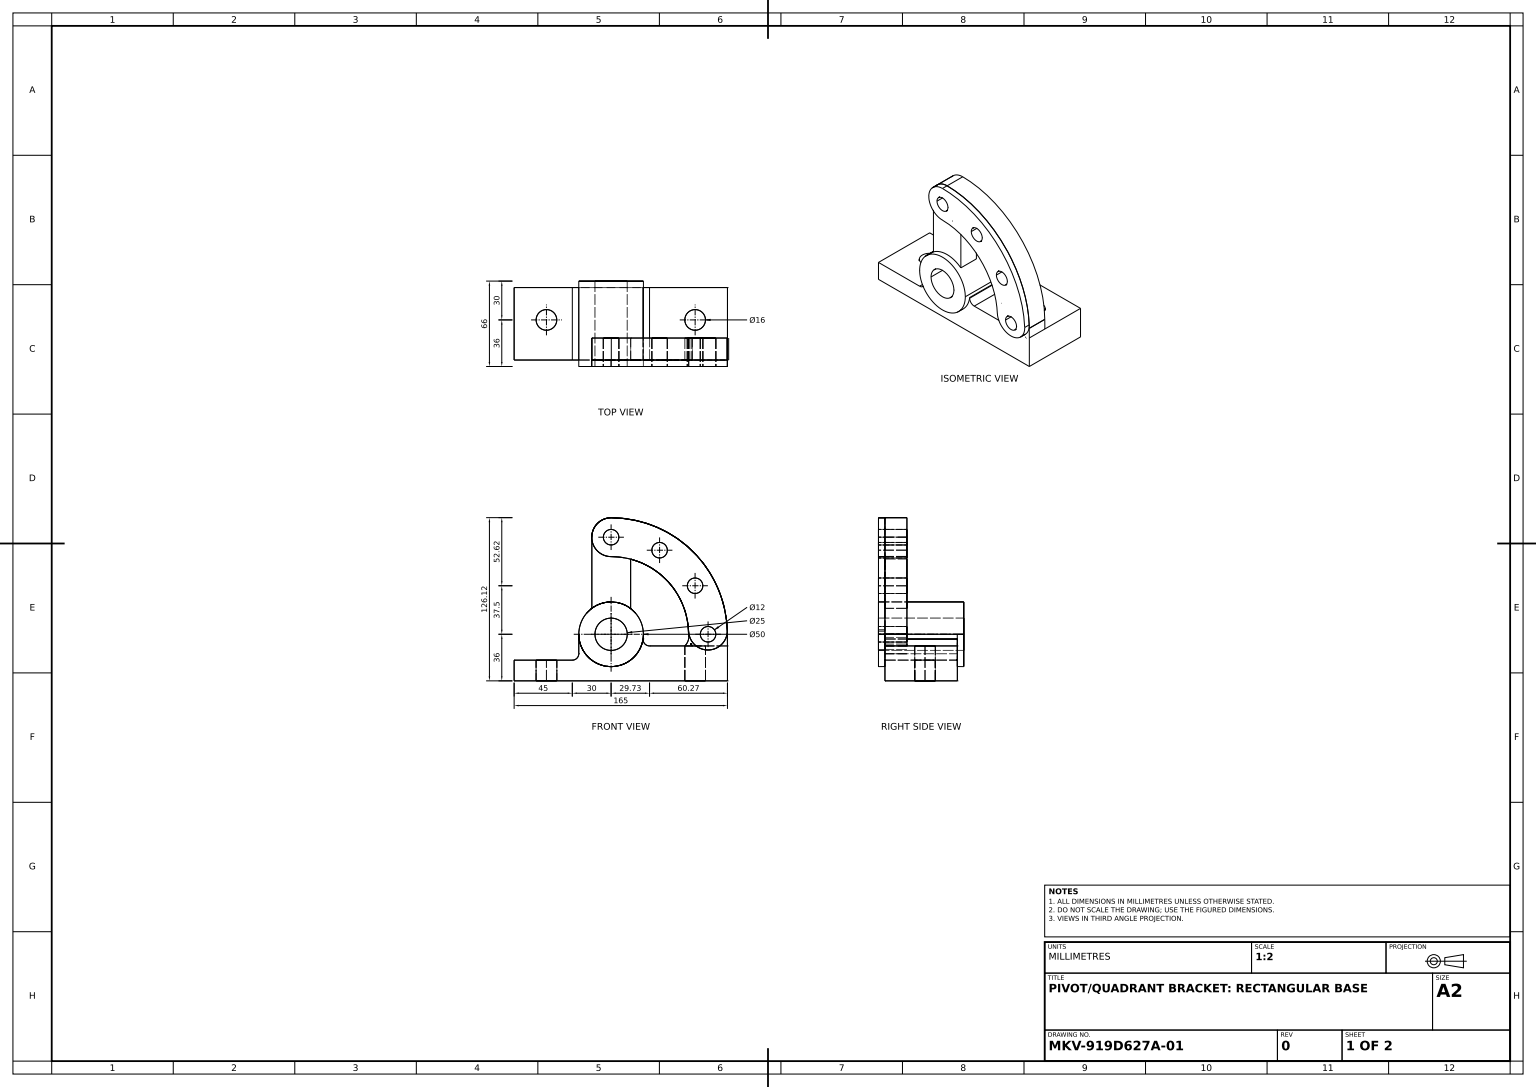
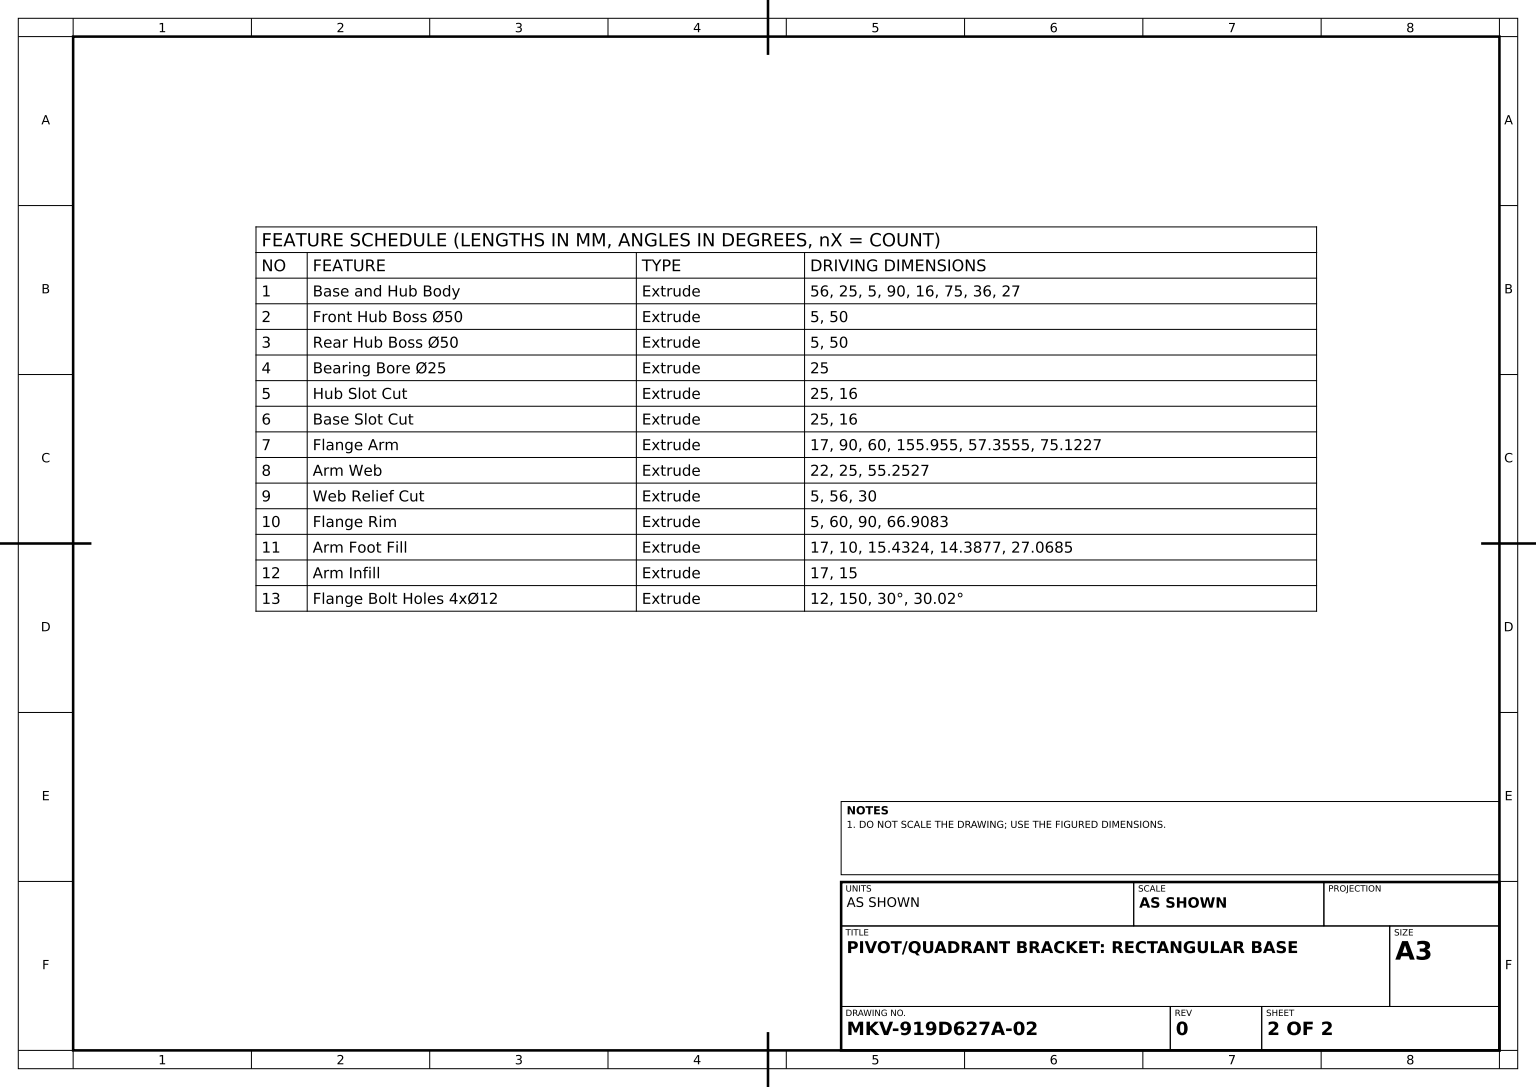
solid
v1 (25,0,-11)
v2 (25,0,5)
e1 v1 v2 CIRCLE(AX(P(25,0,-3),D(0,1,0),D(0,0,1)),8)
e2 v2 v1 CIRCLE(AX(P(25,0,-3),D(0,1,0),D(0,0,1)),8)
v3 (132,0,-3)
v4 (148,0,-3)
e3 v3 v4 CIRCLE(AX(P(140,0,-3),D(0,1,0),D(-1,0,0)),8)
e4 v4 v3 CIRCLE(AX(P(140,0,-3),D(0,1,0),D(-1,0,0)),8)
v5 (0,0,28)
v6 (0,0,-28)
e5 v5 v6 LINE
v7 (165,0,-28)
e6 v6 v7 LINE
v8 (165,0,28)
e7 v8 v7 LINE
e8 v5 v8 LINE
face PLANE(AX(P(0,0,28),D(0,1,0),D(0,0,1))) rev [e1 e2] [e3 e4] [e5 e6 -e7 -e8]
v9 (75,126,33)
v10 (60,111,33)
e9 v9 v10 CIRCLE(AX(P(75,111,33),D(0,0,1),D(1,0,0)),15)
v11 (75,126,28)
e10 v9 v11 LINE
v12 (64.0036439244,121.2019680973,28)
e11 v11 v12 CIRCLE(AX(P(75,111,28),D(0,0,1),D(1,0,0)),15)
v13 (60,111,28)
e12 v12 v13 CIRCLE(AX(P(75,111,28),D(0,0,1),D(1,0,0)),15)
e13 v10 v13 LINE
face CYL(AX(P(75,111,33),D(0,0,-1),D(-1,0,0)),15) [-e9 e10 e11 e12 -e13]
v14 (106.5,100.9519052838,33)
v15 (118.5,100.9519052838,33)
e14 v14 v15 CIRCLE(AX(P(112.5,100.9519052838,33),D(0,0,1),D(1,0,0)),6)
v16 (118.5,100.9519052838,11)
e15 v16 v15 LINE
v17 (106.5,100.9519052838,11)
e16 v17 v16 CIRCLE(AX(P(112.5,100.9519052838,11),D(0,0,1),D(1,0,0)),6)
e17 v17 v14 LINE
face CYL(AX(P(112.5,100.9519052838,-33),D(0,0,1),D(1,0,0)),6) rev [e14 -e15 -e16 e17]
v18 (136.9462929603,28.4158166916,11)
v19 (136.9462929603,28.4158166916,28)
e18 v18 v19 LINE
v20 (137.8192138792,27,28)
e19 v19 v20 CIRCLE(AX(P(150.5000050186,35.7953418305,28),D(0,0,1),D(1,0,0)),15.4324496382)
v21 (137.8192138792,27,11)
e20 v21 v20 LINE
e21 v18 v21 CIRCLE(AX(P(150.5000050186,35.7953418305,11),D(0,0,1),D(1,0,0)),15.4324496382)
face CYL(AX(P(150.5000050186,35.7953418305,11),D(0,0,1),D(1,0,0)),15.4324496382) rev [e18 e19 -e20 -e21]
v22 (60.1126828794,109.1648463416,28)
v23 (60.1126828794,56.0840182471,28)
e22 v22 v23 LINE
v24 (90.1126828794,55.9149897361,28)
e23 v23 v24 CIRCLE(AX(P(75,36,28),D(0,0,-1),D(1,0,0)),25)
v25 (90.1126828794,94.0655389727,28)
e24 v24 v25 LINE
v26 (75,96,28)
e25 v26 v25 CIRCLE(AX(P(75,36,28),D(0,0,-1),D(1,0,0)),60)
e26 v22 v26 CIRCLE(AX(P(75,111,28),D(0,0,1),D(1,0,0)),15)
face PLANE(AX(P(45,21,28),D(0,0,1),D(1,0,0))) [e22 e23 e24 -e25 -e26]
v27 (90.1126828794,94.1593040082,28)
e27 v25 v27 LINE
v28 (90.1126828794,55.9149897361,11)
e28 v28 v24 LINE
v29 (90.1126828794,94.1593040082,11)
e29 v29 v28 LINE
e30 v27 v29 LINE
face PLANE(AX(P(90.1126828794,0,11),D(-1,0,0),D(0,-1,0))) rev [-e27 -e24 -e28 -e29 -e30]
v30 (100,36,-33)
v31 (50,36,-33)
e31 v30 v31 CIRCLE(AX(P(75,36,-33),D(0,0,-1),D(-1,0,0)),25)
e32 v31 v30 CIRCLE(AX(P(75,36,-33),D(0,0,-1),D(-1,0,0)),25)
v32 (87.5,36,-33)
v33 (62.5,36,-33)
e33 v32 v33 CIRCLE(AX(P(75,36,-33),D(0,0,1),D(1,0,0)),12.5)
e34 v33 v32 CIRCLE(AX(P(75,36,-33),D(0,0,1),D(1,0,0)),12.5)
face PLANE(AX(P(75,36,-33),D(0,0,-1),D(-1,0,0))) [e31 e32] [e33 e34]
v34 (141.457402299,96.6911334518,28)
v35 (75.1575772552,126.1226769983,28)
e35 v34 v35 CIRCLE(AX(P(74.8878066875,36.1230813112,28),D(0,0,1),D(1,0,0)),90)
v36 (164.8785967145,37.4106023036,28)
e36 v36 v34 CIRCLE(AX(P(74.8878066875,36.1230813112,28),D(0,0,1),D(1,0,0)),90)
v37 (164.8878066875,36.1230813112,28)
e37 v37 v36 CIRCLE(AX(P(74.8878066875,36.1230813112,28),D(0,0,1),D(1,0,0)),90)
v38 (164.8878066875,36.1230813112,11)
e38 v38 v37 LINE
v39 (75.1575772552,126.1226769983,11)
e39 v38 v39 CIRCLE(AX(P(74.8878066875,36.1230813112,11),D(0,0,1),D(1,0,0)),90)
e40 v39 v35 LINE
face CYL(AX(P(74.8878066875,36.1230813112,11),D(0,0,1),D(1,0,0)),90) [-e35 -e36 -e37 -e38 e39 e40]
v40 (164.8876854953,35.9753837378,28)
e41 v40 v37 CIRCLE(AX(P(74.8878066875,36.1230813112,28),D(0,0,1),D(1,0,0)),90)
v41 (134.9571151191,38.2681152077,28)
e42 v41 v36 CIRCLE(AX(P(149.9463938989,38.8351440097,28),D(0,0,1),D(1,0,0)),15)
v42 (119.2862122558,76.4812475603,28)
e43 v42 v41 CIRCLE(AX(P(75,36,28),D(0,0,-1),D(1,0,0)),60)
v43 (134.8878066875,36.1230813112,28)
e44 v42 v43 CIRCLE(AX(P(74.8878066875,36.1230813112,28),D(0,0,-1),D(1,0,0)),60)
v44 (134.8877258927,36.0246162622,28)
e45 v43 v44 CIRCLE(AX(P(74.8878066875,36.1230813112,28),D(0,0,-1),D(1,0,0)),60)
v45 (135.0895883187,33.5473030871,28)
e46 v44 v45 CIRCLE(AX(P(149.887705694,36,28),D(0,0,1),D(1,0,0)),15)
v46 (132,27,28)
e47 v46 v45 CIRCLE(AX(P(125.1144370231,34.2518289066,28),D(0,0,1),D(1,0,0)),10)
v47 (104.7321374946,27,28)
e48 v46 v47 LINE
v48 (99.7321374946,32,28)
e49 v47 v48 CIRCLE(AX(P(104.7321374946,32,28),D(0,0,-1),D(1,0,0)),5)
v49 (99.7767812455,32.6666666667,28)
e50 v48 v49 CIRCLE(AX(P(104.7321374946,32,28),D(0,0,-1),D(1,0,0)),5)
v50 (50,36,28)
e51 v50 v49 CIRCLE(AX(P(75,36,28),D(0,0,1),D(1,0,0)),25)
v51 (50,21,28)
e52 v50 v51 LINE
v52 (45,16,28)
e53 v51 v52 CIRCLE(AX(P(45,21,28),D(0,0,-1),D(1,0,0)),5)
v53 (0,16,28)
e54 v52 v53 LINE
e55 v53 v5 LINE
v54 (165,27,28)
e56 v8 v54 LINE
e57 v54 v40 LINE
v55 (137.887705694,27,28)
e58 v19 v55 CIRCLE(AX(P(149.887705694,36,28),D(0,0,1),D(1,0,0)),15)
e59 v55 v20 LINE
face PLANE(AX(P(45,21,28),D(0,0,1),D(1,0,0))) [e41 e37 -e42 -e43 e44 e45 e46 -e47 e48 e49 e50 -e51 e52 e53 e54 e55 e8 e56 e57] [-e19 e58 e59]
v56 (132,27,-3)
v57 (148,27,-3)
e60 v56 v57 CIRCLE(AX(P(140,27,-3),D(0,1,0),D(-1,0,0)),8)
e61 v4 v57 LINE
e62 v3 v56 LINE
face CYL(AX(P(140,0,-3),D(0,1,0),D(-1,0,0)),8) rev [e60 -e61 -e3 e62]
v58 (60.1126828794,111.0777826225,11)
v59 (60.1126828794,56.0840182471,11)
e63 v58 v59 LINE
e64 v59 v23 LINE
v60 (60.1126828794,111.0777826225,28)
e65 v60 v22 LINE
e66 v60 v58 LINE
face PLANE(AX(P(60.1126828794,0,11),D(-1,0,0),D(0,0,1))) [e63 e64 -e22 -e65 e66]
v61 (69,111,33)
v62 (81,111,33)
e67 v61 v62 CIRCLE(AX(P(75,111,33),D(0,0,1),D(1,0,0)),6)
v63 (81,111,11)
e68 v63 v62 LINE
v64 (69,111,11)
e69 v64 v63 CIRCLE(AX(P(75,111,11),D(0,0,1),D(1,0,0)),6)
e70 v64 v61 LINE
face CYL(AX(P(75,111,-33),D(0,0,1),D(1,0,0)),6) rev [e67 -e68 -e69 e70]
v65 (25,16,-11)
v66 (25,16,5)
e71 v65 v66 CIRCLE(AX(P(25,16,-3),D(0,1,0),D(0,0,1)),8)
e72 v66 v65 CIRCLE(AX(P(25,16,-3),D(0,1,0),D(0,0,1)),8)
v67 (45,16,-28)
e73 v52 v67 LINE
v68 (0,16,-28)
e74 v67 v68 LINE
e75 v53 v68 LINE
face PLANE(AX(P(0,16,28),D(0,-1,0),D(0,0,-1))) rev [-e71 -e72] [-e54 e73 e74 -e75]
v69 (164.9356726786,39.4021728116,28)
e76 v36 v69 CIRCLE(AX(P(149.9463938989,38.8351440097,28),D(0,0,1),D(1,0,0)),15)
v70 (164.9356726786,39.4021728116,33)
e77 v70 v69 LINE
v71 (134.9571151191,38.2681152077,33)
e78 v71 v70 CIRCLE(AX(P(149.9463938989,38.8351440097,33),D(0,0,1),D(1,0,0)),15)
e79 v71 v41 LINE
face CYL(AX(P(149.9463938989,38.8351440097,33),D(0,0,-1),D(-1,0,0)),15) [e42 e76 -e77 -e78 e79]
e80 v68 v6 LINE
face PLANE(AX(P(0,0,28),D(1,0,0),D(0,0,-1))) rev [e75 e80 -e5 -e55]
v72 (87.5,36,33)
e81 v32 v72 LINE
v73 (62.5,36,33)
e82 v72 v73 CIRCLE(AX(P(75,36,33),D(0,0,1),D(1,0,0)),12.5)
e83 v33 v73 LINE
face CYL(AX(P(75,36,-33),D(0,0,1),D(1,0,0)),12.5) rev [-e33 e81 e82 -e83]
v74 (135.0895883187,33.5473030871,11)
e84 v74 v45 LINE
v75 (132,27,11)
e85 v75 v74 CIRCLE(AX(P(125.1144370231,34.2518289066,11),D(0,0,1),D(1,0,0)),10)
e86 v75 v46 LINE
face CYL(AX(P(125.1144370231,34.2518289066,11),D(0,0,1),D(1,0,0)),10) rev [-e84 -e85 e86 e47]
e87 v69 v34 CIRCLE(AX(P(75,36,28),D(0,0,1),D(1,0,0)),90)
face PLANE(AX(P(112.4731969494,37.4175720048,28),D(0,0,1),D(1,0,0))) rev [-e87 -e76 e36]
v76 (50,36,-28)
v77 (50,21,-28)
e88 v76 v77 LINE
e89 v51 v77 LINE
e90 v50 v76 LINE
face PLANE(AX(P(50,36,28),D(1,0,0),D(0,1,0))) rev [e88 -e89 -e52 e90]
e91 v77 v67 CIRCLE(AX(P(45,21,-28),D(0,0,-1),D(1,0,0)),5)
face CYL(AX(P(45,21,28),D(0,0,-1),D(-1,0,0)),5) rev [e91 -e73 -e53 e89]
e92 v2 v66 LINE
e93 v1 v65 LINE
face CYL(AX(P(25,0,-3),D(0,1,0),D(0,0,1)),8) rev [-e92 -e1 e93 e71]
e94 v34 v11 CIRCLE(AX(P(75,36,28),D(0,0,1),D(1,0,0)),90)
e95 v35 v12 CIRCLE(AX(P(75.1126154939,111.1227443837,28),D(0,0,1),D(1,0,0)),15)
face PLANE(AX(P(45,21,28),D(0,0,1),D(1,0,0))) [-e94 e35 e95 -e11]
e96 v70 v9 CIRCLE(AX(P(75,36,33),D(0,0,1),D(1,0,0)),90)
face CYL(AX(P(75,36,33),D(0,0,-1),D(-1,0,0)),90) [e77 e87 e94 -e10 -e96]
v78 (133.9519052838,73.5,11)
v79 (133.9519052838,73.5,33)
e97 v78 v79 LINE
v80 (145.9519052838,73.5,11)
e98 v80 v78 CIRCLE(AX(P(139.9519052838,73.5,11),D(0,0,1),D(1,0,0)),6)
v81 (145.9519052838,73.5,33)
e99 v80 v81 LINE
e100 v81 v79 CIRCLE(AX(P(139.9519052838,73.5,33),D(0,0,1),D(1,0,0)),6)
face CYL(AX(P(139.9519052838,73.5,-33),D(0,0,1),D(1,0,0)),6) rev [-e97 -e98 e99 e100]
e101 v28 v59 CIRCLE(AX(P(75,36,11),D(0,0,1),D(1,0,0)),25)
v82 (100,36,33)
v83 (50,36,33)
e102 v82 v83 CIRCLE(AX(P(75,36,33),D(0,0,1),D(1,0,0)),25)
e103 v82 v30 LINE
e104 v76 v31 LINE
e105 v83 v50 LINE
face CYL(AX(P(75,36,28),D(0,0,-1),D(-1,0,0)),25) [-e101 e28 -e23 -e64] [-e102 e103 -e32 -e104 -e90 -e105]
v84 (156,36,11)
v85 (156,36,33)
e106 v84 v85 LINE
v86 (144,36,11)
e107 v86 v84 CIRCLE(AX(P(150,36,11),D(0,0,1),D(1,0,0)),6)
v87 (144,36,33)
e108 v86 v87 LINE
e109 v87 v85 CIRCLE(AX(P(150,36,33),D(0,0,1),D(1,0,0)),6)
face CYL(AX(P(150,36,-33),D(0,0,1),D(1,0,0)),6) rev [-e106 -e107 e108 e109]
e110 v60 v12 CIRCLE(AX(P(75.1126154939,111.1227443837,28),D(0,0,-1),D(1,0,0)),15)
e111 v13 v22 CIRCLE(AX(P(75,111,28),D(0,0,1),D(1,0,0)),15)
face PLANE(AX(P(112.4731969494,37.4175720048,28),D(0,0,1),D(1,0,0))) rev [-e110 e65 -e111 -e12]
e112 v83 v82 CIRCLE(AX(P(75,36,33),D(0,0,1),D(1,0,0)),25)
v88 (99.7767812455,32.6666666667,-28)
e113 v49 v88 LINE
e114 v88 v76 CIRCLE(AX(P(75,36,-28),D(0,0,-1),D(-1,0,0)),25)
face CYL(AX(P(75,36,28),D(0,0,-1),D(-1,0,0)),25) [e104 -e31 -e103 -e112 e105 e51 e113 e114]
v89 (99.7321374946,32,-28)
e115 v48 v89 LINE
e116 v89 v88 CIRCLE(AX(P(104.7321374946,32,-28),D(0,0,-1),D(1,0,0)),5)
face CYL(AX(P(104.7321374946,32,28),D(0,0,-1),D(-1,0,0)),5) rev [-e50 e115 e116 -e113]
e117 v73 v72 CIRCLE(AX(P(75,36,33),D(0,0,1),D(1,0,0)),12.5)
face CYL(AX(P(75,36,-33),D(0,0,1),D(1,0,0)),12.5) rev [e83 e117 -e81 -e34]
v90 (104.7321374946,27,-28)
e118 v47 v90 LINE
e119 v90 v89 CIRCLE(AX(P(104.7321374946,32,-28),D(0,0,-1),D(1,0,0)),5)
face CYL(AX(P(104.7321374946,32,28),D(0,0,-1),D(-1,0,0)),5) rev [-e115 -e49 e118 e119]
e120 v78 v80 CIRCLE(AX(P(139.9519052838,73.5,11),D(0,0,1),D(1,0,0)),6)
e121 v79 v81 CIRCLE(AX(P(139.9519052838,73.5,33),D(0,0,1),D(1,0,0)),6)
face CYL(AX(P(139.9519052838,73.5,-33),D(0,0,1),D(1,0,0)),6) rev [-e120 e97 e121 -e99]
e122 v39 v58 CIRCLE(AX(P(75.1126154939,111.1227443837,11),D(0,0,1),D(1,0,0)),15)
face CYL(AX(P(75.1126154939,111.1227443837,11),D(0,0,1),D(1,0,0)),15) [-e95 -e40 e122 -e66 e110]
v91 (137.887705694,27,11)
e123 v18 v91 CIRCLE(AX(P(149.887705694,36,11),D(0,0,1),D(1,0,0)),15)
e124 v55 v91 LINE
face CYL(AX(P(149.887705694,36,11),D(0,0,1),D(1,0,0)),15) [e123 -e124 -e58 -e18]
v92 (134.8878066875,36.1230813112,11)
e125 v92 v43 LINE
v93 (134.8877258927,36.0246162622,11)
e126 v92 v93 CIRCLE(AX(P(74.8878066875,36.1230813112,11),D(0,0,-1),D(1,0,0)),60)
e127 v93 v44 LINE
face CYL(AX(P(74.8878066875,36.1230813112,11),D(0,0,1),D(1,0,0)),60) rev [-e125 e126 e127 -e45]
v94 (165,27,-28)
e128 v94 v90 LINE
e129 v7 v94 LINE
face PLANE(AX(P(45,21,-28),D(0,0,1),D(1,0,0))) rev [-e128 -e129 -e6 -e80 -e74 -e91 -e88 -e114 -e116 -e119]
e130 v29 v92 CIRCLE(AX(P(74.8878066875,36.1230813112,11),D(0,0,-1),D(1,0,0)),60)
e131 v27 v42 CIRCLE(AX(P(74.8878066875,36.1230813112,28),D(0,0,-1),D(1,0,0)),60)
face CYL(AX(P(74.8878066875,36.1230813112,11),D(0,0,1),D(1,0,0)),60) rev [e30 e130 e125 -e44 -e131]
v95 (75,96,33)
e132 v10 v95 CIRCLE(AX(P(75,111,33),D(0,0,1),D(1,0,0)),15)
e133 v95 v71 CIRCLE(AX(P(75,36,33),D(0,0,-1),D(1,0,0)),60)
e134 v62 v61 CIRCLE(AX(P(75,111,33),D(0,0,1),D(1,0,0)),6)
e135 v85 v87 CIRCLE(AX(P(150,36,33),D(0,0,1),D(1,0,0)),6)
e136 v15 v14 CIRCLE(AX(P(112.5,100.9519052838,33),D(0,0,1),D(1,0,0)),6)
face PLANE(AX(P(112.4731969494,37.4175720048,33),D(0,0,1),D(1,0,0))) [e9 e132 e133 e78 e96] [-e100 -e121] [-e67 -e134] [-e109 -e135] [-e14 -e136]
e137 v21 v75 LINE
e138 v93 v74 CIRCLE(AX(P(149.887705694,36,11),D(0,0,1),D(1,0,0)),15)
v96 (164.8876854953,35.9753837378,11)
e139 v96 v38 CIRCLE(AX(P(74.8878066875,36.1230813112,11),D(0,0,1),D(1,0,0)),90)
v97 (165,27,11)
e140 v97 v96 LINE
e141 v97 v91 LINE
e142 v63 v64 CIRCLE(AX(P(75,111,11),D(0,0,1),D(1,0,0)),6)
e143 v16 v17 CIRCLE(AX(P(112.5,100.9519052838,11),D(0,0,1),D(1,0,0)),6)
e144 v84 v86 CIRCLE(AX(P(150,36,11),D(0,0,1),D(1,0,0)),6)
face PLANE(AX(P(112.3877561907,36.0615406556,11),D(0,0,1),D(1,0,0))) rev [e120 e98] [e137 e85 -e138 -e126 -e130 e29 e101 -e63 -e122 -e39 -e139 -e140 e141 -e123 e21] [e69 e142] [e143 e16] [e107 e144]
e145 v95 v26 LINE
face CYL(AX(P(75,111,33),D(0,0,-1),D(-1,0,0)),15) [e26 -e145 -e132 e13 e111]
face CYL(AX(P(25,0,-3),D(0,1,0),D(0,0,1)),8) rev [e92 e72 -e93 -e2]
face CYL(AX(P(75,111,-33),D(0,0,1),D(1,0,0)),6) rev [-e70 -e142 e68 e134]
e146 v97 v94 LINE
e147 v57 v56 CIRCLE(AX(P(140,27,-3),D(0,1,0),D(-1,0,0)),8)
face PLANE(AX(P(165,27,28),D(0,-1,0),D(1,0,0))) rev [-e48 -e86 -e137 e20 -e59 e124 -e141 e146 e128 -e118] [-e60 -e147]
face CYL(AX(P(149.887705694,36,11),D(0,0,1),D(1,0,0)),15) [-e46 -e127 e138 e84]
face CYL(AX(P(140,0,-3),D(0,1,0),D(-1,0,0)),8) rev [e61 e147 -e62 -e4]
e148 v96 v40 LINE
face CYL(AX(P(74.8878066875,36.1230813112,11),D(0,0,1),D(1,0,0)),90) [-e148 e139 e38 -e41]
e149 v54 v97 LINE
face PLANE(AX(P(164.8876854953,35.9753837378,11),D(0.9999217139,0.0125126363,0),D(-0.0125126363,0.9999217139,0))) [e149 e140 e148 -e57]
face CYL(AX(P(112.5,100.9519052838,-33),D(0,0,1),D(1,0,0)),6) rev [e136 -e17 -e143 e15]
face PLANE(AX(P(75,36,33),D(0,0,1),D(1,0,0))) [-e117 -e82] [e112 e102]
face PLANE(AX(P(165,0,28),D(-1,0,0),D(0,-1,0))) rev [-e56 e7 e129 -e146 -e149]
e150 v25 v42 CIRCLE(AX(P(75,36,28),D(0,0,-1),D(1,0,0)),60)
face PLANE(AX(P(112.4731969494,37.4175720048,28),D(0,0,1),D(1,0,0))) rev [e131 -e150 e27]
face CYL(AX(P(75,36,33),D(0,0,-1),D(-1,0,0)),60) rev [e43 -e79 -e133 e145 e25 e150]
face CYL(AX(P(150,36,-33),D(0,0,1),D(1,0,0)),6) rev [-e108 -e144 e106 e135]
